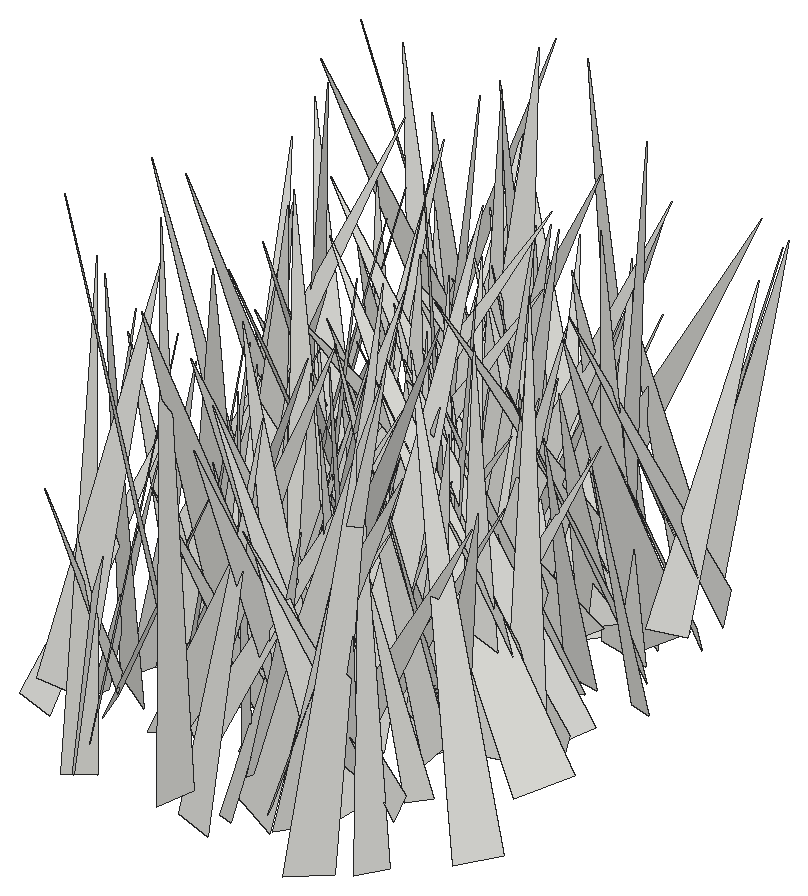
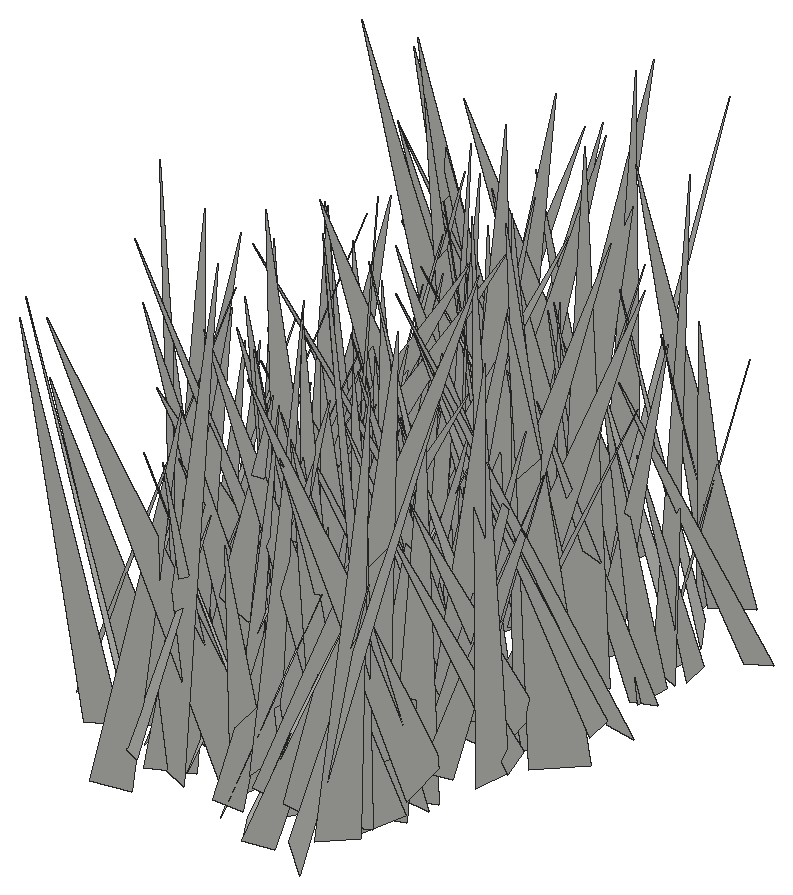
# SketchUp Ruby script. Lengths in inches.
U = 1.inch
M = Sketchup.active_model
def pt(a) = Geom::Point3d.new(a.map { |v| v * U })
def face(e, loops, mat)
  f = e.add_face(loops[0].map { |a| pt(a) })
  loops[1..].each { |l| e.add_face(l.map { |a| pt(a) }).erase! }
  f.material = f.back_material = mat if mat
  f
end
# faces: each face lists its corners as indices into pts; further lists are holes
def faces(e, pts, list, mat = nil) = list.each { |f| face(e, (f[0].is_a?(Array) ? f : [f]).map { |l| l.map { |i| pts[i] } }, mat) }
# xy, xz, yz: faces in a plane at the given z, y or x. An outline is a flat list of corners, or four numbers for a rectangle; further outlines are holes
def ring(l) = l.size == 4 ? [[l[0], l[1]], [l[2], l[1]], [l[2], l[3]], [l[0], l[3]]] : l.each_slice(2).to_a
def flat(e, list, mat, &to3) = list.each { |f| face(e, (f[0].is_a?(Array) ? f : [f]).map { |l| ring(l).map { |u, v| to3.(u, v) } }, mat) }
def xy(e, z, list, mat = nil) = flat(e, list, mat) { |x, y| [x, y, z] }
def xz(e, y, list, mat = nil) = flat(e, list, mat) { |x, z| [x, y, z] }
def yz(e, x, list, mat = nil) = flat(e, list, mat) { |y, z| [x, y, z] }
def lines(e, pts, list) = list.each { |a, b| e.add_line(pt(pts[a]), pt(pts[b])) }
# prism: a flat outline (further loops are holes) pulled along v
def prism(e, loops, v, mat = nil)
  f = face(e, loops, mat); d = Geom::Vector3d.new(v.map { |x| x * U })
  f.pushpull(f.normal.samedirection?(d) ? d.length : -d.length)
end
def box(e, o, s, mat = nil) = prism(e, [[o, [o[0] + s[0], o[1], o[2]], [o[0] + s[0], o[1] + s[1], o[2]], [o[0], o[1] + s[1], o[2]]]], [0, 0, s[2]], mat)
def at(x, y, z, deg = 0) = Geom::Transformation.translation(pt([x, y, z])) * Geom::Transformation.rotation(ORIGIN, Z_AXIS, deg.degrees)
def axes(o, x, y, z) = Geom::Transformation.new([*x, 0, *y, 0, *z, 0, *pt(o).to_a, 1])
def part(name) = M.definitions.add(name)
# library, detail: a bought-in or finely detailed component or shape, given as its bounding box
def library(name, o, s) = part(name).tap { |d| box(d.entities, o, s) }
def detail(e, o, s) = box(e.add_group.entities, o, s)
def put(e, d, t, mat = nil) = e.add_instance(d, t).tap { |i| i.material = mat if mat }
def group(e, t, mat = nil) = e.add_group.tap { |g| g.transformation = t; g.material = mat if mat }.entities
root = M.entities
c1 = part("fur_instance\#9")
p = [[0.8125,0,1.79],[0.67,-0.02,1.48],[0,-0.11,0],[0,0.11,0]]
faces(c1.entities,p,[[0,1,2,3]])
put(root,c1,axes([111.13,127.14,-28.22],[0.30593,5.01742,0.69432],[4.86404,-0.09691,-1.44288],[1.4134,-0.75252,4.8152]))
put(root,c1,axes([114.32,143.77,-28.22],[-5.20648,-5.71637,1.32602],[-5.85189,5.18966,-0.6046],[0.43665,1.3904,7.70836]))
put(root,c1,axes([112.91,139.1875,-27.1],[3.29812,-3.00828,0.87507],[-2.53709,-3.30998,-1.81667],[-1.83812,-0.82908,4.07763]))
put(root,c1,axes([114.51,124.86,-28.22],[-7.06937,0.92542,0.80535],[0.55425,6.6114,-2.73188],[1.09444,2.62944,6.58553]))
put(root,c1,axes([112.12,128.71,-28.22],[3.57631,0.31891,0.97988],[0.16002,-3.66803,0.60973],[-1.01797,0.54376,3.53835]))
put(root,c1,axes([111.04,134.35,-27.1],[4.1398,0.29454,0.02134],[0.28882,-4.10074,0.57065],[-0.06159,0.56772,4.11084]))
put(root,c1,axes([113.52,131.07,-27.1],[-4.62696,1.13691,1.70574],[1.48296,4.76376,0.84751],[1.41525,-1.27471,4.68861]))
put(root,c1,axes([112.28,130.42,-28.22],[4.80103,-0.44543,1.50068],[-0.59366,-4.99749,0.41591],[-1.44845,0.57184,4.80368]))
put(root,c1,axes([110.49,134.09,-27.1],[3.27574,7.01328,0.4286],[6.91428,-3.13335,-1.57325],[1.25002,-1.04703,7.57902]))
put(root,c1,axes([111.65,137.27,-27.1],[4.45385,0.90104,0.34779],[0.77968,-4.32278,1.21461],[-0.57002,1.12752,4.37874]))
put(root,c1,axes([111.55,138.45,-27.1],[7.9282,0.66664,2.15118],[1.11346,-8.00329,-1.62351],[-1.9576,-1.85234,7.78877]))
put(root,c1,axes([113.47,138.57,-27.1],[-0.2394,-4.99537,0.47277],[-5.01072,0.21306,-0.28607],[-0.26442,0.48521,4.99291]))
put(root,c1,axes([112.84,135.41,-27.1],[4.59265,0.40937,1.72839],[-0.43371,-4.3881,2.19176],[-1.72245,2.19644,4.05662]))
put(root,c1,axes([114.52,136.3,-27.1],[-3.46559,5.8146,1.30946],[5.95968,3.40104,0.67057],[0.08042,-1.46897,6.73574]))
put(root,c1,axes([114.18,124.76,-28.22],[3.51213,5.3509,1.08193],[4.75447,-3.63032,2.52063],[-2.68285,0.57134,5.88334]))
put(root,c1,axes([113.43,127.9375,-27.1],[-3.15969,-2.10838,0.70871],[-1.88389,3.19122,1.09464],[1.18257,-0.54957,3.6374]))
put(root,c1,axes([112.76,129.32,-28.22],[-3.13728,-6.42445,2.27927],[-6.51063,3.56742,1.09378],[2.01998,1.52023,7.06539]))
put(root,c1,axes([112.78,143.78,-27.1],[5.63565,-3.00774,1.4531],[-2.80235,-5.80815,-1.15361],[-1.81792,-0.37081,6.28301]))
put(root,c1,axes([112.24,130.87,-28.22],[0.61438,4.77457,1.24038],[4.786,-0.27399,-1.3159],[1.1955,-1.35681,4.63059]))
put(root,c1,axes([113.56,139.31,-28.22],[0.3484,4.1984,0.59349],[4.23915,-0.35779,0.04247],[-0.09183,-0.58788,4.21262]))
put(root,c1,axes([116.55,131.27,-27.1],[-3.06653,-6.21678,2.70439],[-6.51984,1.89062,-3.04678],[-1.85842,3.62531,6.22648]))
put(root,c1,axes([112.43,126.69,-27.1],[-0.87926,6.56228,2.62812],[6.83144,1.46959,-1.38397],[1.81713,-2.34956,6.47466]))
put(root,c1,axes([111.8,135.15,-28.22],[4.60789,-6.31495,1.14074],[-6.41656,-4.51508,0.92427],[0.08686,1.46561,7.76253]))
put(root,c1,axes([114.55,142.6,-27.1],[-3.7389,-0.44853,0.79303],[-0.43438,3.82202,0.11371],[0.80087,-0.02096,3.764]))
put(root,c1,axes([114.84,133.95,-27.1],[-4.29176,-1.39668,0.34406],[-1.22552,4.11722,1.42648],[0.75311,-1.25938,4.28195]))
put(root,c1,axes([113.74,139.13,-28.22],[2.29625,-5.32789,2.30917],[-5.72704,-2.48806,-0.04565],[-0.95905,2.10109,5.80148]))
put(root,c1,axes([113.4,126.79,-28.22],[-4.45958,-2.36263,3.46386],[-3.3219,5.07642,-0.81428],[2.55838,2.47306,4.98064]))
put(root,c1,axes([114.13,141.4375,-28.22],[2.60909,-3.89298,2.22887],[-4.24925,-2.97119,-0.21539],[-1.4377,1.71676,4.68148]))
put(root,c1,axes([113.35,135.02,-28.22],[5.51365,3.20537,1.24598],[2.89904,-5.59864,1.57419],[-1.84998,0.77981,6.18035]))
put(root,c1,axes([115.32,135.375,-27.1],[-0.75565,-7.24529,1.23648],[-7.25287,0.53359,-1.30585],[-1.19119,1.34729,7.16659]))
put(root,c1,axes([114.73,140.34,-27.1],[-4.39266,5.33205,2.64396],[5.82364,4.52851,0.54275],[1.2274,-2.40386,6.88706]))
put(root,c1,axes([115.15,131.24,-27.1],[-6.13848,3.83375,0.83292],[3.60337,6.1212,-1.61832],[1.55148,0.95163,7.05405]))
put(root,c1,axes([115.72,134.93,-28.22],[-3.48001,3.233,0.8636],[3.33945,3.27515,1.19585],[-0.21495,-1.45934,4.59703]))
put(root,c1,axes([115.39,143.04,-27.1],[0.76231,-8.24421,0.75454],[-8.09051,-0.90251,-1.68715],[-1.75496,0.57958,8.10565]))
put(root,c1,axes([112.91,139.73,-27.1],[7.28027,0.47928,1.68125],[-0.05604,-7.13268,2.27604],[-1.74733,2.22571,6.93193]))
put(root,c1,axes([112.79,134.76,-28.22],[1.84601,-7.44066,1.73932],[-7.59322,-1.58595,1.27441],[0.85535,1.97933,7.55956]))
put(root,c1,axes([113.875,140.49,-28.22],[2.77965,-6.05851,0.20454],[-6.05263,-2.78627,-0.276],[-0.3362,0.0706,6.66001]))
put(root,c1,axes([112.9,132.76,-27.1],[1.80193,-7.44469,0.50754],[-7.36471,-1.69029,1.35351],[1.20089,0.80465,7.53912]))
put(root,c1,axes([116.74,126.82,-27.1],[-6.42891,-4.93695,1.78859],[-5.18873,6.40682,-0.96596],[0.80598,1.86616,8.04806]))
put(root,c1,axes([114.52,135.54,-28.22],[0.72086,7.11073,0.81641],[7.15729,-0.71063,-0.13028],[0.04812,-0.82534,7.14599]))
put(root,c1,axes([112.81,128.33,-28.22],[4.64757,1.11707,0.03174],[1.0994,-4.54603,-0.98676],[0.20042,-0.96672,4.67697]))
put(root,c1,axes([114.93,138.99,-27.1],[3.23703,-3.40023,0.62778],[-3.13183,-3.24768,-1.44163],[-1.46538,-0.57015,4.46784]))
put(root,c1,axes([116.51,143.17,-28.22],[-3.58425,-2.16039,0.18109],[-2.16614,3.55434,-0.47063],[-0.08907,0.49634,4.15845]))
put(root,c1,axes([115.57,143.81,-28.22],[3.91388,-2.85851,1.41513],[-2.09693,-3.9939,-2.26798],[-2.40345,-1.17037,4.2832]))
put(root,c1,axes([115.57,141.73,-28.22],[2.36967,1.89121,2.13493],[2.35412,-2.86396,-0.07595],[-1.61018,-1.40392,3.03088]))
put(root,c1,axes([116.12,134.01,-27.1],[0.1057,3.9764,0.92499],[3.9126,-0.36287,1.11284],[-1.16573,-0.85739,3.81897]))
put(root,c1,axes([115.86,131.43,-28.22],[-0.09942,-3.58739,1.13729],[-3.70553,-0.10534,-0.65623],[-0.65715,1.13676,3.52826]))
put(root,c1,axes([115.7,138.4375,-27.1],[-3.21539,5.33291,0.27404],[5.21793,3.20577,-1.16191],[1.13501,0.36996,6.11789]))
put(root,c1,axes([115.09,128.65,-27.1],[4.32331,2.64676,1.47041],[2.57631,-4.56233,0.63737],[-1.59061,-0.19566,5.02892]))
put(root,c1,axes([114.86,136.15,-27.1],[-2.17172,3.54056,2.13295],[3.72846,2.71807,-0.7156],[1.78427,-1.37037,4.09143]))
put(root,c1,axes([114.55,141.65,-27.1],[3.71133,-3.4553,1.19556],[-3.62183,-3.7076,0.52772],[-0.50083,1.20708,5.04327]))
put(root,c1,axes([114.375,139.39,-27.1],[1.48764,5.46016,1.29529],[5.56167,-1.25605,-1.09283],[0.74757,-1.52092,5.55267]))
put(root,c1,axes([115.63,128.68,-28.22],[2.58353,5.00263,1.49189],[5.09313,-2.78069,0.50442],[-1.14546,-1.08079,5.60772]))
put(root,c1,axes([115.18,137.09,-28.22],[-3.16063,-7.46069,0.64697],[-7.21635,3.22195,1.90087],[2.00118,-0.16476,7.87643]))
put(root,c1,axes([116.06,129.37,-27.1],[-2.49672,2.92464,0.96124],[2.97957,2.60694,-0.1927],[0.77439,-0.6012,3.84057]))
put(root,c1,axes([115.46,131.65,-27.1],[5.32876,3.34285,1.26399],[2.90072,-5.37113,1.97605],[-2.08763,1.0697,5.97207]))
put(root,c1,axes([117.55,142.85,-28.22],[-3.47734,-1.80435,0.22841],[-1.8088,3.48242,-0.02761],[0.19,0.12974,3.9175]))
put(root,c1,axes([116.81,128.91,-27.1],[-4.46885,1.59045,1.08144],[1.18804,4.43404,-1.61169],[1.51249,1.21632,4.46123]))
put(root,c1,axes([119.71,138.625,-28.22],[-6.653,2.83628,0.09553],[2.75112,6.38619,1.99099],[-0.69638,-1.86767,6.95291]))
put(root,c1,axes([115.68,134.17,-28.22],[6.26441,4.08516,1.86388],[4.05019,-6.52197,0.68206],[-1.9387,-0.42509,7.44756]))
put(root,c1,axes([118.77,136.1875,-28.22],[-4.69197,-2.31538,0.05263],[-2.28134,4.60011,-1.00642],[-0.39908,0.92541,5.13447]))
put(root,c1,axes([115.78,131.07,-27.1],[5.60712,-6.07402,0.33398],[-5.83929,-5.5015,-2.02021],[-1.70529,-1.13347,8.01575]))
put(root,c1,axes([115.56,138.64,-28.22],[4.80804,6.17674,2.98381],[6.78482,-4.81897,-0.95722],[-1.01068,-2.96612,7.76873]))
put(root,c1,axes([113.63,140.9,-28.22],[6.68383,-3.60485,0.36068],[-3.59385,-6.50181,1.61538],[0.45749,1.59067,7.42019]))
put(root,c1,axes([114.31,130.19,-27.1],[6.51578,-0.90085,0.09034],[-0.89347,-6.50413,-0.41604],[-0.1463,-0.39981,6.56459]))
put(root,c1,axes([117.01,141.72,-27.1],[-6.68895,-1.28776,2.75903],[-1.15,7.23488,0.5888],[2.81923,-0.10417,6.78629]))
put(root,c1,axes([113.76,137.35,-27.1],[3.2036,5.15972,0.63397],[4.7617,-2.61371,-2.78969],[2.08586,-1.95793,5.39475]))
put(root,c1,axes([117.02,129.625,-27.1],[-4.18199,-2.55213,0.91155],[-1.98836,4.02848,2.15666],[1.84139,-1.44616,4.39901]))
put(root,c1,axes([115.4,134.9,-28.22],[3.31192,-3.28223,0.0309],[-3.2384,-3.26025,0.79144],[0.53549,0.5836,4.59516]))
put(root,c1,axes([118.64,123.85,-27.1],[-8.04005,-0.21045,2.18635],[-0.63833,8.16213,-1.56173],[2.10165,1.67397,7.88972]))
put(root,c1,axes([117.91,141.38,-27.1],[-3.18277,2.93848,0.48438],[2.88307,3.21784,-0.5768],[0.74643,0.10079,4.29324]))
put(root,c1,axes([116.41,134.31,-27.1],[4.19181,1.99584,0.5753],[1.88629,-4.2003,0.82769],[-0.86965,0.50967,4.56832]))
put(root,c1,axes([115.87,141.87,-28.22],[3.91302,0.34843,0.25725],[0.41449,-3.69091,-1.30566],[-0.12562,-1.32482,3.70519]))
put(root,c1,axes([113.78,134.36,-27.1],[4.07618,6.66518,0.05677],[6.29765,-3.82934,-2.59208],[2.18344,-1.39809,7.37028]))
put(root,c1,axes([117.63,142.57,-28.22],[0.4513,-4.46287,0.47479],[-4.46772,-0.49211,-0.3789],[-0.42669,0.43236,4.4696]))
put(root,c1,axes([118.41,138.375,-28.22],[0.17252,3.92598,1.26935],[3.97591,-0.49782,0.99933],[-1.10305,-1.18034,3.80058]))
put(root,c1,axes([118.74,140.39,-27.1],[-5.92753,-0.80933,1.51712],[-1.07571,5.99367,-1.00549],[1.34146,1.2301,5.89742]))
put(root,c1,axes([118.84,126.79,-28.22],[2.66286,4.62658,1.9724],[4.32664,-3.24515,1.77077],[-2.56433,-0.67099,5.03592]))
put(root,c1,axes([117.11,135.67,-28.22],[-4.12278,4.06528,3.37823],[4.64279,4.83304,-0.14992],[2.52655,-2.24755,5.78803]))
put(root,c1,axes([116.05,140.95,-27.1],[3.45559,-4.90486,0.92565],[-4.98413,-3.32981,0.96246],[0.2699,1.30779,5.9222]))
put(root,c1,axes([117.0625,135.16,-28.22],[4.3108,-3.69492,0.61953],[-3.55093,-4.33068,-1.12044],[-1.19463,-0.46051,5.56597]))
put(root,c1,axes([116.33,131.0625,-27.1],[-3.15581,4.82371,2.67558],[4.59437,4.00448,-1.80054],[3.05265,-1.04019,5.47589]))
put(root,c1,axes([117.66,138.52,-28.22],[-2.49427,4.27012,1.59064],[4.35584,2.76683,-0.59729],[1.33819,-1.04698,4.90903]))
put(root,c1,axes([118.45,130.14,-27.1],[5.58768,-4.04107,3.86555],[-4.58295,-6.44048,-0.10822],[-3.20457,2.16447,6.89498]))
put(root,c1,axes([117.23,139.37,-27.1],[-5.12716,5.45276,3.67809],[5.84452,5.9162,-0.62364],[3.01704,-2.19425,7.45865]))
put(root,c1,axes([117.73,133.69,-28.22],[0.74131,3.87524,0.12897],[3.87698,-0.74271,0.03187],[-0.05555,-0.12068,3.94537]))
put(root,c1,axes([119.35,136.43,-28.22],[-7.86516,0.65945,1.92725],[0.13584,7.83978,-2.12819],[2.03241,2.02799,7.60042]))
put(root,c1,axes([116.71,133.55,-27.1],[-2.8265,-4.26887,1.57231],[-3.66111,3.23328,2.19698],[2.70032,-0.08465,4.62446]))
put(root,c1,axes([118.23,131.5,-28.22],[4.04445,-6.42376,0.8146],[-6.13253,-4.10829,-1.94934],[-2.07854,-0.37835,7.33638]))
put(root,c1,axes([120.5625,137.57,-28.22],[-2.09774,5.99421,0.07606],[5.73274,1.98235,1.88224],[-1.75272,-0.69034,6.06533]))
put(root,c1,axes([121.17,132.25,-28.22],[-4.9129,-5.75828,0.52895],[-5.68371,4.68095,-1.83254],[-1.06438,1.58274,7.34412]))
put(root,c1,axes([117.79,130.98,-28.22],[0.58274,-3.68979,0.92218],[-3.78198,-0.46356,0.53511],[0.40205,0.98748,3.697]))
put(root,c1,axes([117.77,130.84,-27.1],[1.5026,-5.2869,1.47769],[-5.48951,-1.44343,0.41772],[0.01326,1.53554,5.48039]))
put(root,c1,axes([119.35,136.23,-28.22],[-4.95355,2.49117,1.9463],[2.93301,4.97148,1.10159],[1.17959,-1.90003,5.43416]))
put(root,c1,axes([119.15,134.51,-28.22],[-0.20928,5.81187,1.2771],[5.90875,0.05179,0.73257],[-0.70395,-1.2931,5.76932]))
put(root,c1,axes([119.64,139.67,-28.22],[-5.02237,2.51021,1.68016],[2.86774,4.98644,1.12241],[0.94877,-1.78398,5.50142]))
put(root,c1,axes([118.8,135.43,-28.22],[2.12896,3.50938,0.78952],[3.35263,-2.26833,1.04217],[-1.30344,-0.10245,3.97015]))
put(root,c1,axes([120.03,141.4,-28.22],[-3.2308,-2.41105,0.08917],[-2.40238,3.20101,-0.49122],[-0.22293,0.4467,4.00124]))
put(root,c1,axes([118.82,140.12,-27.1],[-3.91635,-3.27614,1.36892],[-3.24396,4.13005,0.60351],[1.44353,0.39293,5.07017]))
put(root,c1,axes([119.95,135.55,-28.22],[-3.93894,0.78438,0.2139],[0.7314,3.88076,-0.76228],[0.35506,0.70765,3.94328]))
put(root,c1,axes([120.91,136.71,-28.22],[-3.24563,2.42896,0.17461],[2.25293,2.88449,1.75171],[-0.92447,-1.49811,3.65588]))
put(root,c1,axes([119.4,135.31,-27.1],[3.60121,-2.60608,3.3834],[-3.59297,-4.24118,0.55747],[-2.30861,2.53545,4.41017]))
put(root,c1,axes([116.37,126.66,-27.1],[6.24865,-3.61776,1.18124],[-3.80474,-5.99015,1.78079],[-0.08657,2.13519,6.99733]))
put(root,c1,axes([116.14,134.625,-28.22],[3.95823,-3.37287,0.12226],[-3.1364,-3.60629,2.0534],[1.24667,1.63622,4.7778]))
put(root,c1,axes([119.01,128.5625,-28.22],[4.85297,5.01471,2.08252],[4.89411,-5.24941,1.23566],[-2.35199,-0.5761,6.86817]))
put(root,c1,axes([120.69,139.48,-28.22],[-4.49285,4.90641,0.97236],[5.00159,4.41981,0.80831],[0.04935,-1.26349,6.60342]))
put(root,c1,axes([118.97,131.05,-28.22],[-0.85461,3.70026,0.75554],[3.7566,0.91253,-0.21994],[0.38824,-0.68446,3.79129]))
put(root,c1,axes([118.68,137.32,-27.1],[-3.43446,-5.67079,0.15135],[-5.3482,3.29577,2.1239],[1.89143,-0.97791,6.28032]))
put(root,c1,axes([119.51,133.34,-27.1],[-4.59387,1.36569,1.34916],[1.20913,4.77619,-0.71765],[1.49109,0.33451,4.73854]))
put(root,c1,axes([119.14,125.39,-28.22],[4.44404,5.53922,0.27989],[5.13876,-4.2472,2.46279],[-2.08674,1.3376,6.66087]))
put(root,c1,axes([117.33,133.91,-27.1],[2.31038,-4.41979,0.71264],[-4.3801,-2.06578,1.38834],[0.92579,1.25629,4.79008]))
put(root,c1,axes([117.9,138.08,-27.1],[1.20072,-3.47995,0.99765],[-3.52529,-0.88496,1.15597],[0.82322,1.28603,3.49507]))
put(root,c1,axes([118.26,138.5,-28.22],[3.89931,-1.45547,0.98195],[-1.58431,-3.9476,0.44006],[-0.75669,0.76505,4.13877]))
put(root,c1,axes([116.29,132.75,-28.22],[8.18505,-1.50624,0.16494],[-1.43272,-7.98824,-1.85106],[-0.49323,-1.79175,8.11402]))
put(root,c1,axes([118.68,124.58,-28.22],[1.78136,5.8506,1.71123],[6.09225,-1.76893,-0.29408],[-0.20572,-1.72409,6.10871]))
put(root,c1,axes([120.58,133.23,-27.1],[-3.8761,2.85036,0.12124],[2.83481,3.87102,-0.37744],[0.32105,0.23257,4.79648]))
put(root,c1,axes([121.63,137.7,-27.1],[2.28844,-6.77562,0.58153],[-5.77223,-2.2597,-3.61376],[-3.59563,-0.68473,6.17144]))
put(root,c1,axes([118.23,138.33,-28.22],[6.38697,-1.69717,1.73981],[-1.81592,-6.58358,0.24416],[-1.61547,0.69051,6.6041]))
put(root,c1,axes([117.84,138.21,-28.22],[4.9565,-0.0282,0.53243],[-0.1703,-4.80111,1.33099],[-0.50525,1.34155,4.77453]))
put(root,c1,axes([120.18,142.09,-28.22],[-2.90002,-7.26429,3.03178],[-7.85451,2.88308,-0.60516],[0.51793,3.0479,7.79832]))
put(root,c1,axes([117.67,140.65,-28.22],[4.04604,3.23344,0.3968],[3.2461,-3.94826,-0.92578],[0.27467,-0.96906,5.09593]))
put(root,c1,axes([119.46,129.31,-28.22],[5.40513,-4.44008,1.03103],[-3.91993,-5.34397,-2.46351],[-2.32626,-1.31164,6.54682]))
put(root,c1,axes([118.18,140.68,-28.22],[3.59656,-0.31618,0.04156],[-0.31764,-3.59357,0.14939],[-0.02828,0.15246,3.60734]))
put(root,c1,axes([119.76,140.43,-28.22],[0.83118,5.18677,1.07004],[5.28228,-0.88982,0.21009],[-0.38088,-1.02179,5.24874]))
put(root,c1,axes([120.54,127.32,-27.1],[-3.35147,5.54659,2.9979],[6.27053,3.28643,0.92965],[0.65767,-3.06906,6.41348]))
put(root,c1,axes([121.12,132.89,-27.1],[-6.29577,-3.22015,2.48262],[-3.79064,6.30377,-1.43636],[1.47099,2.46225,6.92409]))
put(root,c1,axes([120.27,143.54,-27.1],[-1.91573,-3.10975,0.18965],[-3.07242,1.92263,0.49017],[0.51647,-0.09744,3.61944]))
put(root,c1,axes([121.97,133.72,-27.1],[-4.83845,-0.36416,0.05457],[-0.36621,4.6838,-1.21411],[-0.03844,1.21473,4.69778]))
put(root,c1,axes([120.6,134.05,-28.22],[-6.51752,1.2418,2.00991],[0.54856,6.53189,-2.25684],[2.29801,1.9627,6.23913]))
put(root,c1,axes([119.9375,133.6875,-27.1],[-0.22883,-5.12281,0.23524],[-5.12454,0.23734,0.18366],[0.19416,0.22665,5.12463]))
put(root,c1,axes([120.32,133.4,-27.1],[3.4021,4.35261,1.87369],[4.47593,-3.70904,0.48912],[-1.55627,-1.15238,5.50275]))
put(root,c1,axes([118.2,140,-27.1],[6.4862,-0.82849,0.61771],[-0.87391,-6.49276,0.46816],[-0.55158,0.54452,6.52212]))
put(root,c1,axes([120.54,135.12,-27.1],[-2.95191,2.4359,0.97471],[2.3622,3.10602,-0.60836],[1.1418,-0.12828,3.77853]))
put(root,c1,axes([117.35,126.46,-27.1],[4.17015,5.48726,0.52169],[5.30168,-3.81404,-2.26221],[1.50809,-1.76505,6.51019]))
put(root,c1,axes([120.72,129.1,-27.1],[-6.29891,4.40553,1.36932],[3.82289,6.28157,-2.62437],[2.58248,1.44677,7.22479]))
put(root,c1,axes([117.67,138.24,-27.1],[3.41975,6.53108,1.33927],[6.45057,-2.86091,-2.51965],[1.68487,-2.30293,6.92828]))
put(root,c1,axes([124.83,132.17,-28.22],[-5.23637,6.32875,0.17784],[5.87309,4.76933,3.20385],[-2.36465,-2.16904,7.5636]))
put(root,c1,axes([118.68,127.28,-27.1],[2.58495,3.56171,0.23056],[3.43761,-2.40789,-1.34382],[0.96012,-0.96809,4.1907]))
put(root,c1,axes([119.54,126.52,-27.1],[4.26328,-1.39926,0.74192],[-1.39292,-4.32659,-0.15583],[-0.75375,0.08115,4.48433]))
put(root,c1,axes([121.29,131.51,-28.22],[-3.58724,1.8714,1.40372],[2.1412,3.66165,0.59026],[0.94225,-1.19623,4.00275]))
put(root,c1,axes([120.11,142.03,-28.22],[4.15376,-5.21591,0.7578],[-5.12927,-4.22232,-0.94677],[-1.21268,-0.00681,6.60024]))
put(root,c1,axes([119.57,131.01,-27.1],[3.16954,2.48643,0.53995],[2.54162,-3.13416,-0.48689],[-0.1185,-0.71733,3.99891]))
put(root,c1,axes([119.95,136.63,-27.1],[3.72524,-2.31212,0.81738],[-2.32656,-3.80205,-0.15146],[-0.77532,0.29988,4.38182]))
put(root,c1,axes([121.03,128.83,-28.22],[3.99412,4.65299,3.2629],[5.30006,-4.48907,-0.08624],[-2.05092,-2.53923,6.13155]))
put(root,c1,axes([120.68,128.8,-27.1],[5.22033,-0.21574,2.13038],[0.1303,-5.5713,-0.88347],[-2.13731,-0.86658,5.14955]))
put(root,c1,axes([120.87,143.74,-28.22],[1.67149,-5.33301,0.8085],[-5.34441,-1.75188,-0.5067],[-0.72935,0.6152,5.5658]))
put(root,c1,axes([122.06,136.71,-28.22],[-0.32554,-5.06602,0.7464],[-4.99056,0.14633,-1.18345],[-1.14716,0.80105,4.9366]))
put(root,c1,axes([120.08,134.51,-28.22],[5.34451,-1.51745,2.02584],[-2.07356,-5.33917,1.4711],[-1.45157,2.03988,5.35746]))
put(root,c1,axes([117.65,141.42,-28.22],[5.9864,-4.39629,0.74457],[-4.35138,-5.48795,2.58196],[0.97326,2.50473,6.96403]))
put(root,c1,axes([122.85,126.22,-27.1],[-6.22259,1.31552,1.1088],[1.51746,6.15727,1.21077],[0.81078,-1.42761,6.24382]))
put(root,c1,axes([121.6,141.22,-28.22],[-6.50454,-4.83681,0.42708],[-4.2184,5.98256,3.50717],[2.40464,-2.5885,7.30777]))
put(root,c1,axes([123.7,134.86,-28.22],[-4.61226,3.61546,0.79034],[3.61757,4.1381,2.18138],[-0.78062,-2.18488,5.43931]))
put(root,c1,axes([121.12,135.32,-27.1],[5.49101,0.89671,2.25711],[-0.37206,-5.20349,2.97239],[-2.40004,2.85822,4.70322]))
put(root,c1,axes([122.63,130.27,-27.1],[-6.25427,-0.78477,1.30734],[-0.71032,6.38344,0.43371],[1.34924,-0.27711,6.28838]))
put(root,c1,axes([118.12,129.58,-27.1],[8.10386,-2.02713,0.06413],[-2.02706,-8.10412,-0.01624],[-0.06615,-0.00019,8.35354]))
put(root,c1,axes([118.1,128.34,-28.22],[2.55754,-6.5759,0.86107],[-6.14173,-2.00015,2.96707],[2.50263,1.81158,6.40156]))
put(root,c1,axes([119.6,126.04,-28.22],[2.9133,6.77269,2.26525],[7.08174,-2.424,-1.8604],[0.9217,-2.7826,7.13411]))
put(root,c1,axes([121.02,125,-27.1],[4.46685,2.95329,0.59597],[2.75098,-4.43263,1.34675],[-1.2285,0.81223,5.18275]))
put(root,c1,axes([121.82,138.72,-27.1],[4.3952,-2.19196,2.60814],[-2.70598,-4.83259,0.49862],[-2.06997,1.6632,4.88608]))
put(root,c1,axes([119.8,130.14,-28.22],[4.70172,-1.10111,0.26171],[-1.12934,-4.49092,1.39405],[0.07438,1.41645,4.62334]))
put(root,c1,axes([122.38,131.54,-28.22],[-3.88391,-3.01754,1.00768],[-2.99103,4.00531,0.46572],[1.08383,0.24005,4.89626]))
put(root,c1,axes([121.28,138.87,-27.1],[1.53045,-4.60076,0.23907],[-4.60681,-1.52625,0.11946],[0.03806,0.26453,4.84716]))
put(root,c1,axes([119.63,134.84,-28.22],[2.74788,4.31889,0.7575],[4.17328,-2.30167,-2.01583],[1.34551,-1.68135,4.70533]))
put(root,c1,axes([121.27,131.46,-27.1],[3.01124,-3.84874,1.35887],[-4.04465,-3.04041,0.35153],[-0.54781,1.29229,4.87409]))
put(root,c1,axes([122.63,129.48,-28.22],[1.65267,-3.08975,1.39314],[-3.11179,-1.99748,-0.7386],[-1.34319,0.82596,3.42525]))
put(root,c1,axes([123.75,127.24,-27.1],[-4.70083,-1.74871,0.0814],[-1.70109,4.61801,0.97093],[0.41342,-0.88228,4.92068]))
put(root,c1,axes([119.69,129.42,-28.22],[4.10331,-3.61689,0.17449],[-3.47529,-3.85943,1.7253],[1.0172,1.40442,5.19061]))
put(root,c1,axes([122.78,139.02,-28.22],[-3.83453,-4.44323,0.31037],[-4.29048,3.7947,1.3169],[1.19597,-0.63261,5.71941]))
put(root,c1,axes([122.39,132.47,-28.22],[-1.61639,5.70202,2.80279],[6.31476,1.76115,0.05886],[0.70173,-2.71416,5.92641]))
put(root,c1,axes([121.59,139.53,-27.1],[-3.32783,-6.52848,3.29816],[-6.89122,4.01297,0.99019],[2.45153,2.41834,7.26051]))
put(root,c1,axes([121.89,139.31,-28.22],[-0.4517,-7.27096,2.0225],[-7.50286,0.65147,0.6664],[0.81515,1.96726,7.25444]))
put(root,c1,axes([121.97,137.34,-28.22],[0.02895,-4.95019,0.58964],[-4.94989,0.0415,0.59139],[0.59214,0.58889,4.91483]))
put(root,c1,axes([124.1,125.58,-28.22],[-5.96382,1.04535,0.88629],[0.82737,5.90096,-1.39268],[1.09259,1.23747,5.8924]))
put(root,c1,axes([123.51,133.04,-27.1],[-0.65155,5.99766,1.58433],[6.18323,0.49957,0.65163],[-0.49968,-1.63861,5.99765]))
put(root,c1,axes([122.21,124.66,-27.1],[6.62959,-1.41825,2.66639],[-1.99694,-6.88369,1.30369],[-2.26567,1.91728,6.65307]))
put(root,c1,axes([123.03,141.16,-28.22],[-2.38013,-2.88459,0.25848],[-2.75196,2.35686,0.96161],[0.90246,-0.42079,3.61403]))
put(root,c1,axes([123.94,134.24,-28.22],[-4.07436,-2.22938,0.28557],[-2.14023,4.02883,0.91657],[0.68639,-0.67121,4.55307]))
put(root,c1,axes([122.33,140.44,-28.22],[5.40488,-4.57462,0.50738],[-4.27322,-5.27816,-2.06831],[-1.71004,-1.26929,6.77215]))
put(root,c1,axes([123.74,141.46,-27.1],[-5.24067,-3.21189,0.67738],[-2.84495,5.08085,2.08111],[1.63749,-1.45206,5.78359]))
put(root,c1,axes([122.16,126.76,-27.1],[1.97582,-3.11414,0.08334],[-3.10691,-1.9626,0.3224],[0.22782,0.24287,3.67393]))
put(root,c1,axes([124.13,122.8,-27.1],[-7.73799,2.57835,1.8542],[1.9672,7.72518,-2.53263],[2.4932,1.90688,7.75308]))
put(root,c1,axes([122.02,142.65,-27.1],[0.68635,-5.64905,2.27441],[-5.90756,-0.06201,1.6287],[1.47832,2.3749,5.45254]))
put(root,c1,axes([125.98,127.86,-28.22],[-6.63605,2.7216,0.19643],[2.70208,6.62626,-0.52374],[0.38006,0.41041,7.15332]))
put(root,c1,axes([121.78,141.75,-27.1],[5.2265,3.38981,1.10604],[3.55749,-5.09026,-1.20993],[-0.2416,-1.62138,6.11091]))
put(root,c1,axes([122.125,131.45,-27.1],[0.90872,-5.0896,0.45336],[-4.90772,-0.74115,1.51668],[1.42262,0.69427,4.94262]))
put(root,c1,axes([124.2,137.14,-28.22],[-1.30736,-3.53096,1.01989],[-3.67333,1.2908,-0.2398],[0.12042,1.04076,3.75757]))
put(root,c1,axes([123.33,139.36,-27.1],[-3.03856,4.16793,1.35783],[3.96538,3.31773,-1.3102],[1.86846,-0.26309,4.98878]))
